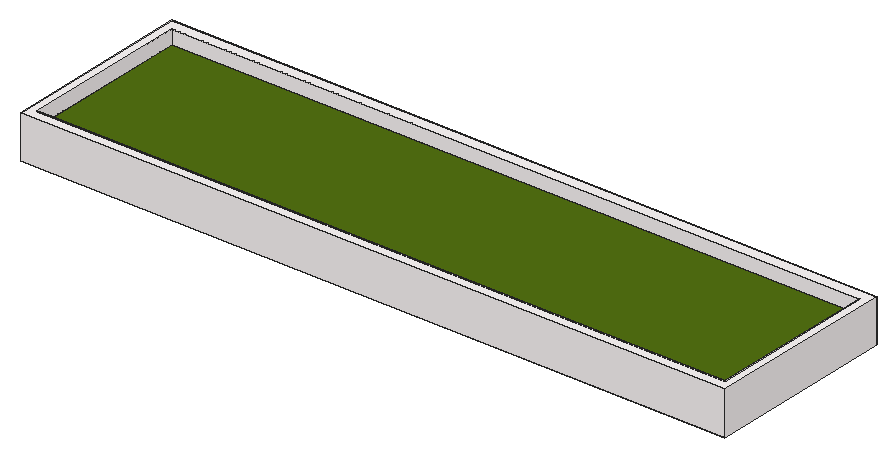
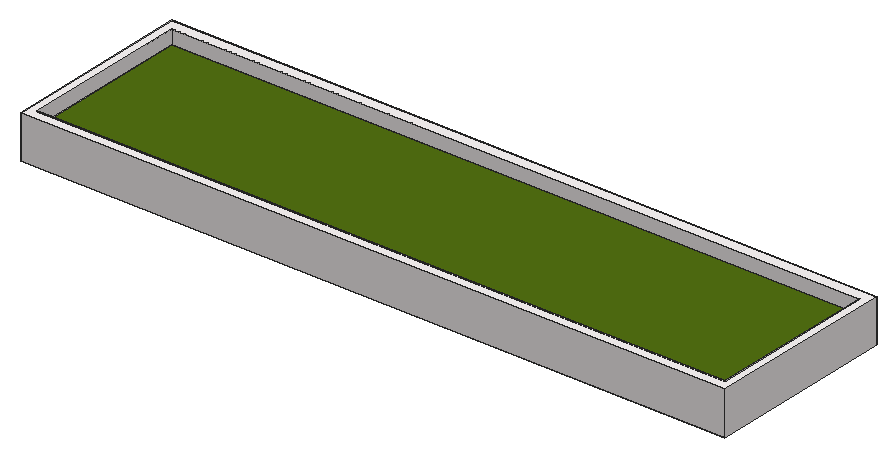
# SketchUp Ruby script. Lengths in inches.
U = 1.inch
M = Sketchup.active_model
def pt(a) = Geom::Point3d.new(a.map { |v| v * U })
def face(e, loops, mat)
  f = e.add_face(loops[0].map { |a| pt(a) })
  loops[1..].each { |l| e.add_face(l.map { |a| pt(a) }).erase! }
  f.material = f.back_material = mat if mat
  f
end
# faces: each face lists its corners as indices into pts; further lists are holes
def faces(e, pts, list, mat = nil) = list.each { |f| face(e, (f[0].is_a?(Array) ? f : [f]).map { |l| l.map { |i| pts[i] } }, mat) }
# xy, xz, yz: faces in a plane at the given z, y or x. An outline is a flat list of corners, or four numbers for a rectangle; further outlines are holes
def ring(l) = l.size == 4 ? [[l[0], l[1]], [l[2], l[1]], [l[2], l[3]], [l[0], l[3]]] : l.each_slice(2).to_a
def flat(e, list, mat, &to3) = list.each { |f| face(e, (f[0].is_a?(Array) ? f : [f]).map { |l| ring(l).map { |u, v| to3.(u, v) } }, mat) }
def xy(e, z, list, mat = nil) = flat(e, list, mat) { |x, y| [x, y, z] }
def xz(e, y, list, mat = nil) = flat(e, list, mat) { |x, z| [x, y, z] }
def yz(e, x, list, mat = nil) = flat(e, list, mat) { |y, z| [x, y, z] }
def lines(e, pts, list) = list.each { |a, b| e.add_line(pt(pts[a]), pt(pts[b])) }
# prism: a flat outline (further loops are holes) pulled along v
def prism(e, loops, v, mat = nil)
  f = face(e, loops, mat); d = Geom::Vector3d.new(v.map { |x| x * U })
  f.pushpull(f.normal.samedirection?(d) ? d.length : -d.length)
end
def box(e, o, s, mat = nil) = prism(e, [[o, [o[0] + s[0], o[1], o[2]], [o[0] + s[0], o[1] + s[1], o[2]], [o[0], o[1] + s[1], o[2]]]], [0, 0, s[2]], mat)
def at(x, y, z, deg = 0) = Geom::Transformation.translation(pt([x, y, z])) * Geom::Transformation.rotation(ORIGIN, Z_AXIS, deg.degrees)
def axes(o, x, y, z) = Geom::Transformation.new([*x, 0, *y, 0, *z, 0, *pt(o).to_a, 1])
def part(name) = M.definitions.add(name)
# library, detail: a bought-in or finely detailed component or shape, given as its bounding box
def library(name, o, s) = part(name).tap { |d| box(d.entities, o, s) }
def detail(e, o, s) = box(e.add_group.entities, o, s)
def put(e, d, t, mat = nil) = e.add_instance(d, t).tap { |i| i.material = mat if mat }
def group(e, t, mat = nil) = e.add_group.tap { |g| g.transformation = t; g.material = mat if mat }.entities
root = M.entities
M.materials.add("[0010_Snow]").color = [255, 250, 250]
M.materials.add("[Vegetation_Blur7]").color = [83, 114, 18]
xy(root,137.875,[[196.21,202.65,279.94,223.21]])
xy(root,137.875,[[[195.23,201.43,280.92,224.43],[196.21,202.65,279.94,223.21]]],"[0010_Snow]")
xy(root,141.36,[[196.21,202.65,279.94,223.21]],"[Vegetation_Blur7]")
xy(root,143.11,[[[195.23,201.43,280.92,224.43],[196.21,202.65,279.94,223.21]]],"[0010_Snow]")
xz(root,201.43,[[195.23,137.875,280.92,143.11]],"[0010_Snow]")
xz(root,202.65,[[196.21,137.875,279.94,141.36],[196.21,141.36,279.94,143.11]],"[0010_Snow]")
xz(root,223.21,[[196.21,137.875,279.94,141.36],[196.21,141.36,279.94,143.11]],"[0010_Snow]")
xz(root,224.43,[[195.23,137.875,280.92,143.11]],"[0010_Snow]")
yz(root,195.23,[[201.43,137.875,224.43,143.11]],"[0010_Snow]")
yz(root,196.21,[[202.65,137.875,223.21,141.36],[202.65,141.36,223.21,143.11]],"[0010_Snow]")
yz(root,279.94,[[202.65,137.875,223.21,141.36],[202.65,141.36,223.21,143.11]],"[0010_Snow]")
yz(root,280.92,[[201.43,137.875,224.43,143.11]],"[0010_Snow]")
